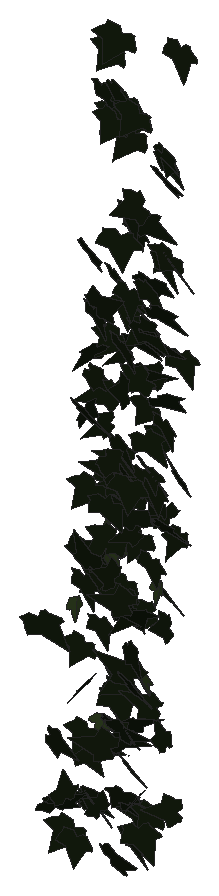
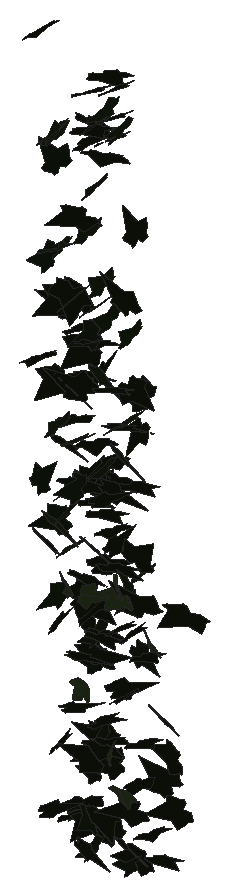
# SketchUp Ruby script. Lengths in inches.
U = 1.inch
M = Sketchup.active_model
def pt(a) = Geom::Point3d.new(a.map { |v| v * U })
def face(e, loops, mat)
  f = e.add_face(loops[0].map { |a| pt(a) })
  loops[1..].each { |l| e.add_face(l.map { |a| pt(a) }).erase! }
  f.material = f.back_material = mat if mat
  f
end
# faces: each face lists its corners as indices into pts; further lists are holes
def faces(e, pts, list, mat = nil) = list.each { |f| face(e, (f[0].is_a?(Array) ? f : [f]).map { |l| l.map { |i| pts[i] } }, mat) }
# xy, xz, yz: faces in a plane at the given z, y or x. An outline is a flat list of corners, or four numbers for a rectangle; further outlines are holes
def ring(l) = l.size == 4 ? [[l[0], l[1]], [l[2], l[1]], [l[2], l[3]], [l[0], l[3]]] : l.each_slice(2).to_a
def flat(e, list, mat, &to3) = list.each { |f| face(e, (f[0].is_a?(Array) ? f : [f]).map { |l| ring(l).map { |u, v| to3.(u, v) } }, mat) }
def xy(e, z, list, mat = nil) = flat(e, list, mat) { |x, y| [x, y, z] }
def xz(e, y, list, mat = nil) = flat(e, list, mat) { |x, z| [x, y, z] }
def yz(e, x, list, mat = nil) = flat(e, list, mat) { |y, z| [x, y, z] }
def lines(e, pts, list) = list.each { |a, b| e.add_line(pt(pts[a]), pt(pts[b])) }
# prism: a flat outline (further loops are holes) pulled along v
def prism(e, loops, v, mat = nil)
  f = face(e, loops, mat); d = Geom::Vector3d.new(v.map { |x| x * U })
  f.pushpull(f.normal.samedirection?(d) ? d.length : -d.length)
end
def box(e, o, s, mat = nil) = prism(e, [[o, [o[0] + s[0], o[1], o[2]], [o[0] + s[0], o[1] + s[1], o[2]], [o[0], o[1] + s[1], o[2]]]], [0, 0, s[2]], mat)
def at(x, y, z, deg = 0) = Geom::Transformation.translation(pt([x, y, z])) * Geom::Transformation.rotation(ORIGIN, Z_AXIS, deg.degrees)
def axes(o, x, y, z) = Geom::Transformation.new([*x, 0, *y, 0, *z, 0, *pt(o).to_a, 1])
def part(name) = M.definitions.add(name)
# library, detail: a bought-in or finely detailed component or shape, given as its bounding box
def library(name, o, s) = part(name).tap { |d| box(d.entities, o, s) }
def detail(e, o, s) = box(e.add_group.entities, o, s)
def put(e, d, t, mat = nil) = e.add_instance(d, t).tap { |i| i.material = mat if mat }
def group(e, t, mat = nil) = e.add_group.tap { |g| g.transformation = t; g.material = mat if mat }.entities
root = M.entities
M.materials.add("1026 AP 7946 SUNNY SIDE UP").color = [254, 231, 186]
M.materials.add("efeu1").color = [18, 25, 13]
M.materials.add("efeu2").color = [43, 57, 29]
c1 = part("ivyleaf_9")
p = [[1.54,2.16,1.25],[1.36,2.04,1.19],[-0.21,0.99,0.68],[-0.71,1.11,0.82],[-0.85,0.86,0.67],[-0.8,0.17,0.21],
  [-0.9,-0.01,0.1],[-0.67,-0.16,-0.02],[-0.08,-0.08,-0.05],[-0.03,-0.6,-0.4],[0.65,-0.88,-0.66],[0.83,-0.6,-0.49],
  [1.29,-0.42,-0.43],[1.8125,-0.07,-0.26],[1.21,0.44,0.15]]
faces(c1.entities,p,[[0,1,2,3,4,5,6,7,8,9,10,11,12,13,14]],"efeu1")
c2 = part("ivyleaf_10")
p = [[0,0.5,-0.03],[-0.0625,2.02,-0.43],[-0.19,2.01,-0.46],[-0.54,1.05,-0.29],[-0.52,0.625,-0.18],[-0.83,0.76,-0.28],
  [-1.16,0.64,-0.33],[-1.15,0.33,-0.24],[-0.77,-0.39,0.02],[-0.3,-0.51,0.16],[0.04,-0.48,0.23],[-0.02,2.01,-0.4375],
  [-0.06,2.01,-0.43],[0.04,-0.49,0.23],[0.67,-0.49,0.14],[1.38,0.36,-0.2],[1.375,0.51,-0.24],[0.81,0.65,-0.19],
  [0.62,0.59,-0.15],[0.6,1.09,-0.28],[0.5,1.23,-0.31]]
faces(c2.entities,p,[[0,1,2,3,4,5,6,7,8,9,10],[11,12,0,13,14,15,16,17,18,19,20]],"efeu2")
put(root,c1,axes([158.63,211.54,302.26],[-0.193,-0.26427,0.31382],[-0.1872,-0.28213,-0.30173],[0.60773,-0.17083,0.00672]),"1026 AP 7946 SUNNY SIDE UP")
put(root,c2,axes([158.375,210.39,301.5],[0.42687,-0.15206,0.25288],[0.29351,-0.16617,-0.31858],[0.34792,0.32675,-0.04151]),"1026 AP 7946 SUNNY SIDE UP")
put(root,c1,axes([158.41,212,299.85],[0.01882,-0.38523,-0.02316],[0.02092,0.0207,-0.39668],[0.60622,0.01125,0.01441]),"1026 AP 7946 SUNNY SIDE UP")
put(root,c1,axes([158.69,212.3,302.82],[-0.28644,-0.2369,0.26948],[-0.16087,-0.24784,-0.30452],[0.53273,-0.20222,0.05294]),"1026 AP 7946 SUNNY SIDE UP")
put(root,c1,axes([158.25,211.11,303.38],[-0.21833,0.04861,0.46385],[0.68202,-0.12015,0.15055],[0.20327,0.45533,-0.00691]),"1026 AP 7946 SUNNY SIDE UP")
put(root,c1,axes([158.86,211.15,313.33],[-0.11675,0.23223,-0.37078],[0.11206,-0.35484,-0.25218],[-0.66589,-0.10043,0.02257]),"1026 AP 7946 SUNNY SIDE UP")
put(root,c2,axes([158.7,211.875,295.34],[0.58802,-0.08102,-0.01424],[-0.03376,-0.03635,-0.39224],[0.12463,0.37243,-0.03908]),"1026 AP 7946 SUNNY SIDE UP")
put(root,c1,axes([158.88,209.57,291.28],[-0.57783,-0.27939,0.06227],[-0.03498,-0.07276,-0.47382],[0.44865,-0.36551,0.04325]),"1026 AP 7946 SUNNY SIDE UP")
put(root,c1,axes([158.34,211,292.09],[0.07738,-0.03027,-0.41689],[0.57726,0.17661,0.03343],[0.27125,-0.36722,0.04778]),"1026 AP 7946 SUNNY SIDE UP")
put(root,c1,axes([158.59,208.22,292.99],[0.03194,0.21488,-0.37217],[0.05224,0.36095,0.22447],[0.66053,-0.03894,0.00024]),"1026 AP 7946 SUNNY SIDE UP")
put(root,c1,axes([158.45,207.96,301.77],[-0.15051,-0.16287,-0.45828],[0.45024,0.34048,-0.1903],[0.5917,-0.30051,0.02824]),"1026 AP 7946 SUNNY SIDE UP")
put(root,c1,axes([158.53,211.29,312.04],[0.41783,-0.28482,-0.21877],[-0.06016,0.23882,-0.38081],[0.55386,0.24081,0.12368]),"1026 AP 7946 SUNNY SIDE UP")
put(root,c1,axes([158.44,211.3,294.39],[0.17299,0.02961,-0.40987],[0.25652,0.37347,0.07726],[0.57276,-0.17621,0.08919]),"1026 AP 7946 SUNNY SIDE UP")
put(root,c1,axes([158.32,208.93,295.69],[0.23693,-0.10053,-0.43884],[0.68673,0.05347,0.14666],[0.02879,-0.44813,0.11315]),"1026 AP 7946 SUNNY SIDE UP")
put(root,c1,axes([158.95,212.25,327.11],[-0.32567,-0.34648,0.24732],[-0.09059,-0.24388,-0.41187],[0.65838,-0.20495,0.06567]),"1026 AP 7946 SUNNY SIDE UP")
put(root,c1,axes([158.59,211.96,325.28],[0.29329,-0.43856,0.06183],[0.01223,-0.06457,-0.491],[0.69646,0.18582,-0.01741]),"1026 AP 7946 SUNNY SIDE UP")
put(root,c2,axes([158.92,211.92,304.68],[0.34785,-0.31239,0.12953],[0.12229,-0.10116,-0.39491],[0.51626,0.23445,0.00627]),"1026 AP 7946 SUNNY SIDE UP")
put(root,c1,axes([159.44,210.62,291.91],[-0.14083,0.19922,0.36869],[-0.32922,0.29125,-0.22],[-0.55173,-0.22464,0.03717]),"1026 AP 7946 SUNNY SIDE UP")
put(root,c1,axes([158.62,211.16,291.87],[0.38671,-0.30197,0.12438],[0.08809,-0.11194,-0.40097],[0.50475,0.2509,-0.02531]),"1026 AP 7946 SUNNY SIDE UP")
put(root,c1,axes([159.15,212.26,313.55],[-0.54377,-0.25492,0.10138],[-0.02444,-0.14234,-0.43062],[0.4298,-0.33061,0.10378]),"1026 AP 7946 SUNNY SIDE UP")
put(root,c1,axes([159.12,210.15,310.93],[-0.01963,-0.03637,-0.45503],[-0.38355,0.36924,-0.02207],[0.58144,0.24234,-0.02992]),"1026 AP 7946 SUNNY SIDE UP")
put(root,c2,axes([158.88,212.37,297.2],[0.01369,-0.1646,0.35889],[0.3275,-0.2922,-0.14891],[0.51127,0.19159,0.08577]),"1026 AP 7946 SUNNY SIDE UP")
put(root,c1,axes([159.19,212.39,327.8],[-0.51356,-0.34852,0.03525],[-0.01394,-0.04125,-0.4918],[0.55078,-0.32601,0.02042]),"1026 AP 7946 SUNNY SIDE UP")
put(root,c1,axes([159.53,211.33,311.34],[-0.5998,-0.0659,0.21862],[-0.27498,-0.17219,-0.37926],[0.21648,-0.40131,0.12398]),"1026 AP 7946 SUNNY SIDE UP")
put(root,c1,axes([159.09,211.98,307.13],[-0.1604,-0.40179,-0.05294],[0.05111,0.04234,-0.42626],[0.63442,-0.105,0.02096]),"1026 AP 7946 SUNNY SIDE UP")
put(root,c1,axes([159.6,211.07,310.07],[-0.58894,0.23093,-0.06474],[0.05545,-0.06464,-0.45215],[-0.37276,-0.37447,0.03503]),"1026 AP 7946 SUNNY SIDE UP")
put(root,c1,axes([158.99,211.19,303.44],[0.15722,-0.36313,0.14132],[0.04607,-0.13632,-0.38874],[0.60979,0.10392,-0.00707]),"1026 AP 7946 SUNNY SIDE UP")
put(root,c1,axes([159.14,210.08,294.875],[0.08827,-0.30312,-0.29422],[-0.06454,0.28101,-0.31584],[0.64981,0.06908,0.0086]),"1026 AP 7946 SUNNY SIDE UP")
put(root,c1,axes([159.02,210.84,315.33],[0.18899,-0.38492,0.19557],[0.07457,-0.18631,-0.4164],[0.67226,0.12888,-0.00879]),"1026 AP 7946 SUNNY SIDE UP")
put(root,c1,axes([159.61,210.33,303.88],[-0.02952,0.29119,0.35933],[-0.01604,0.34708,-0.29847],[-0.71228,-0.01989,-0.00817]),"1026 AP 7946 SUNNY SIDE UP")
put(root,c2,axes([159.26,211.375,303.78],[-0.58108,-0.04479,-0.15772],[0.24827,-0.05235,-0.37779],[0.03286,-0.39647,0.06531]),"1026 AP 7946 SUNNY SIDE UP")
put(root,c1,axes([159.45,209.62,300.22],[-0.35046,-0.32212,0.08648],[-0.05212,-0.08125,-0.40356],[0.52155,-0.22457,0.01777]),"1026 AP 7946 SUNNY SIDE UP")
put(root,c1,axes([159.07,212.1,316.59],[0.32032,-0.37201,0.15364],[0.08346,-0.14317,-0.43725],[0.62591,0.20947,-0.02032]),"1026 AP 7946 SUNNY SIDE UP")
put(root,c1,axes([159.51,211.81,324.42],[-0.3479,-0.32593,0.25349],[-0.08426,-0.25631,-0.39793],[0.63836,-0.21146,0.08562]),"1026 AP 7946 SUNNY SIDE UP")
put(root,c1,axes([159.87,211.92,308.03],[-0.24814,0.02532,0.40139],[-0.5265,-0.22464,-0.12604],[0.31534,-0.35515,0.10541]),"1026 AP 7946 SUNNY SIDE UP")
put(root,c1,axes([159.72,212.05,302.14],[-0.52849,-0.19742,-0.04179],[0.08586,-0.01551,-0.39944],[0.30469,-0.33805,0.04008]),"1026 AP 7946 SUNNY SIDE UP")
put(root,c1,axes([159.66,209.58,296.22],[-0.35773,-0.3412,0.09139],[-0.04162,-0.09105,-0.42203],[0.55355,-0.22735,0.02733]),"1026 AP 7946 SUNNY SIDE UP")
put(root,c1,axes([160.24,210.86,308.13],[-0.23737,-0.08883,-0.43787],[-0.61434,-0.16734,0.17822],[-0.29614,0.41835,-0.01874]),"1026 AP 7946 SUNNY SIDE UP")
put(root,c1,axes([159.91,211.04,304.75],[-0.65537,-0.20291,0.09581],[-0.09333,-0.09165,-0.47469],[0.33912,-0.41736,0.05452]),"1026 AP 7946 SUNNY SIDE UP")
put(root,c1,axes([159.92,209.41,304.24],[0.31097,-0.12589,0.40136],[-0.35368,0.32904,0.22867],[-0.53922,-0.28842,0.08148]),"1026 AP 7946 SUNNY SIDE UP")
put(root,c1,axes([159.55,212.07,297.22],[-0.4124,-0.21599,-0.24334],[0.33465,0.1083,-0.34664],[0.374,-0.33507,0.04184]),"1026 AP 7946 SUNNY SIDE UP")
put(root,c1,axes([159.89,209.7,307.84],[-0.5317,-0.2693,0.06036],[-0.0392,-0.06489,-0.44426],[0.43209,-0.33726,0.03398]),"1026 AP 7946 SUNNY SIDE UP")
put(root,c1,axes([159.46,211.61,325.78],[0.45203,-0.3755,-0.05241],[-0.04078,0.04153,-0.48693],[0.59399,0.28861,0.00645]),"1026 AP 7946 SUNNY SIDE UP")
put(root,c1,axes([159.8,212.25,315.46],[-0.355,-0.35977,-0.0765],[0.18185,0.0107,-0.42736],[0.54759,-0.2368,0.09233]),"1026 AP 7946 SUNNY SIDE UP")
put(root,c2,axes([160.18,212.28,303.92],[0.03925,0.12472,-0.39158],[-0.41255,-0.28331,-0.11496],[-0.47625,0.25569,0.06731]),"1026 AP 7946 SUNNY SIDE UP")
put(root,c1,axes([159.59,207.71,293.53],[0.50354,0.273,-0.06243],[0.03838,0.06684,0.43243],[0.43857,-0.31929,0.03383]),"1026 AP 7946 SUNNY SIDE UP")
put(root,c1,axes([159.95,211.5625,302],[-0.47227,-0.25188,-0.12074],[0.18292,0.04041,-0.40126],[0.39564,-0.31934,0.04139]),"1026 AP 7946 SUNNY SIDE UP")
put(root,c1,axes([160.17,211.51,297.84],[-0.3568,-0.2409,0.29076],[-0.26265,-0.23088,-0.34108],[0.52284,-0.28038,0.02708]),"1026 AP 7946 SUNNY SIDE UP")
put(root,c1,axes([159.81,211.4,297.1],[-0.17577,-0.40182,-0.17373],[0.14838,0.14527,-0.42594],[0.66754,-0.13809,0.04893]),"1026 AP 7946 SUNNY SIDE UP")
put(root,c1,axes([159.76,209.23,303.61],[0.12373,-0.44724,0.05971],[0.00576,-0.06077,-0.46812],[0.70962,0.07847,-0.00661]),"1026 AP 7946 SUNNY SIDE UP")
put(root,c1,axes([159.92,208.56,291.62],[-0.19855,-0.41088,0.013],[0.01253,-0.01809,-0.44273],[0.64637,-0.12586,0.01258]),"1026 AP 7946 SUNNY SIDE UP")
put(root,c1,axes([160.39,211.41,313.63],[-0.51044,0.29772,-0.08286],[0.05277,-0.08443,-0.4525],[-0.48275,-0.32403,0.03815]),"1026 AP 7946 SUNNY SIDE UP")
put(root,c1,axes([159.91,212.03,325.11],[-0.05848,-0.44968,0.12789],[-0.018,-0.12618,-0.46558],[0.73439,-0.0389,-0.00123]),"1026 AP 7946 SUNNY SIDE UP")
put(root,c1,axes([159.62,211,295.98],[0.60817,-0.18434,0.13725],[0.16459,-0.09138,-0.4404],[0.3186,0.3991,-0.03449]),"1026 AP 7946 SUNNY SIDE UP")
put(root,c1,axes([160.15,210.875,324.78],[-0.33681,-0.36204,0.20359],[-0.04085,-0.21265,-0.42716],[0.64883,-0.20132,0.07879]),"1026 AP 7946 SUNNY SIDE UP")
put(root,c1,axes([159.65,209.16,311.61],[0.42336,-0.26869,0.27556],[0.29462,-0.19306,-0.39298],[0.52021,0.328,-0.0017]),"1026 AP 7946 SUNNY SIDE UP")
put(root,c1,axes([159.88,211.27,309.29],[0.32178,-0.37709,-0.02551],[-0.03349,0.01417,-0.44174],[0.59306,0.2054,-0.01111]),"1026 AP 7946 SUNNY SIDE UP")
put(root,c1,axes([160.31,211.18,307.1],[-0.52555,-0.292,0.05395],[-0.02519,-0.06349,-0.456],[0.46625,-0.33257,0.03618]),"1026 AP 7946 SUNNY SIDE UP")
put(root,c1,axes([159.8,210.11,316.07],[-0.08219,0.08953,0.47743],[0.45704,-0.36061,0.10355],[0.58376,0.29494,-0.01385]),"1026 AP 7946 SUNNY SIDE UP")
put(root,c1,axes([159.86,209.45,318.91],[-0.0135,-0.14126,0.46461],[0.27791,-0.42015,-0.13432],[0.69049,0.16634,0.06315]),"1026 AP 7946 SUNNY SIDE UP")
put(root,c1,axes([159.9,212.01,315.68],[0.60451,-0.22304,-0.0106],[-0.02468,-0.00909,-0.45765],[0.35013,0.38445,-0.01396]),"1026 AP 7946 SUNNY SIDE UP")
put(root,c1,axes([160.82,212.23,300.95],[-0.51775,0.0027,0.2258],[-0.33419,-0.10062,-0.32826],[0.08425,-0.38253,0.08555]),"1026 AP 7946 SUNNY SIDE UP")
put(root,c1,axes([160.46,211.85,324.67],[-0.45312,-0.36949,0.04683],[-0.0037,-0.05832,-0.48181],[0.58577,-0.28619,0.03318]),"1026 AP 7946 SUNNY SIDE UP")
put(root,c1,axes([160.51,212.08,304.58],[-0.56101,-0.17067,-0.11801],[0.20164,-0.00792,-0.40277],[0.25151,-0.37435,0.05968]),"1026 AP 7946 SUNNY SIDE UP")
put(root,c1,axes([160.28,210.16,309.07],[0.1949,-0.17801,-0.37693],[-0.06107,0.37456,-0.19965],[0.63544,0.0906,0.09643]),"1026 AP 7946 SUNNY SIDE UP")
put(root,c1,axes([161.04,211.46,291.98],[-0.11962,-0.0545,-0.41965],[-0.63848,-0.05195,0.08505],[-0.09661,0.41082,-0.04244]),"1026 AP 7946 SUNNY SIDE UP")
put(root,c1,axes([160.2,211.36,301.78],[0.41289,-0.36831,0.0219],[-0.01136,-0.03379,-0.46545],[0.58018,0.26145,-0.0247]),"1026 AP 7946 SUNNY SIDE UP")
put(root,c1,axes([160.78,210.6,293.14],[0.31485,0.16325,-0.30777],[-0.34998,-0.2009,-0.26713],[-0.40675,0.29923,-0.00838]),"1026 AP 7946 SUNNY SIDE UP")
put(root,c1,axes([160.39,211.46,316.44],[-0.02217,-0.43747,0.09574],[-0.00509,-0.09537,-0.45147],[0.70404,-0.01446,-0.00025]),"1026 AP 7946 SUNNY SIDE UP")
put(root,c1,axes([160.77,208.23,299.48],[-0.31218,0.28077,-0.26012],[0.1835,-0.22757,-0.35433],[-0.56645,-0.22846,0.02858]),"1026 AP 7946 SUNNY SIDE UP")
put(root,c1,axes([161.11,211.07,305.45],[-0.56809,0.17957,0.01605],[-0.03969,-0.01815,-0.41478],[-0.28049,-0.36112,0.02619]),"1026 AP 7946 SUNNY SIDE UP")
put(root,c1,axes([160.74,212.39,310.66],[-0.32708,-0.29019,0.23698],[-0.00625,-0.2638,-0.34562],[0.58385,-0.16539,0.12906]),"1026 AP 7946 SUNNY SIDE UP")
put(root,c1,axes([160.46,211.25,295.96],[0.27411,0.30839,-0.21995],[0.12762,0.20081,0.36528],[0.57741,-0.19078,0.02368]),"1026 AP 7946 SUNNY SIDE UP")
put(root,c1,axes([161.08,210.99,307.27],[-0.49193,-0.24362,0.14795],[-0.13758,-0.12242,-0.4071],[0.42403,-0.32235,0.03956]),"1026 AP 7946 SUNNY SIDE UP")
put(root,c1,axes([160.66,210.25,295.8],[0.0357,0.12748,-0.43743],[0.06803,0.42323,0.13553],[0.69487,-0.04798,0.00921]),"1026 AP 7946 SUNNY SIDE UP")
put(root,c1,axes([161.13,210.86,324.42],[-0.69989,-0.11343,-0.09335],[0.15094,-0.01349,-0.47182],[0.17042,-0.45391,0.03452]),"1026 AP 7946 SUNNY SIDE UP")
put(root,c1,axes([160.6875,211.51,319.64],[0.0441,-0.36264,0.27513],[0.12083,-0.26188,-0.37331],[0.69972,0.06808,0.04712]),"1026 AP 7946 SUNNY SIDE UP")
put(root,c1,axes([160.78,211.33,314.43],[0.68454,0.09484,0.01284],[0.03144,-0.03596,-0.45743],[-0.14698,0.43402,-0.03803]),"1026 AP 7946 SUNNY SIDE UP")
put(root,c1,axes([161.38,206,295.2],[-0.54665,0.17372,-0.20011],[-0.24649,0.12135,0.39952],[0.32879,0.37981,-0.0332]),"1026 AP 7946 SUNNY SIDE UP")
put(root,c1,axes([161.14,210.53,307.81],[0.47376,-0.21202,0.21313],[-0.19645,0.17845,0.37473],[-0.4238,-0.31974,0.06455]),"1026 AP 7946 SUNNY SIDE UP")
put(root,c1,axes([160.86,209.34,307.62],[-0.2579,-0.23807,-0.32875],[0.36647,0.22061,-0.29292],[0.50545,-0.28143,0.04464]),"1026 AP 7946 SUNNY SIDE UP")
put(root,c1,axes([161.18,210.62,292.73],[0.13548,0.20324,0.34143],[0.14289,0.31832,-0.22436],[-0.59279,0.12318,0.02395]),"1026 AP 7946 SUNNY SIDE UP")
put(root,c1,axes([161.21,210.24,312.43],[-0.09334,-0.0181,0.48812],[-0.32298,-0.42951,-0.04592],[0.67216,-0.2089,0.04572]),"1026 AP 7946 SUNNY SIDE UP")
put(root,c1,axes([161.22,211.81,317.1],[0.57907,0.12079,-0.27461],[-0.3756,-0.12537,-0.39821],[-0.26756,0.43741,-0.03534]),"1026 AP 7946 SUNNY SIDE UP")
put(root,c1,axes([161.52,211.03,312.85],[-0.5695,-0.14385,0.22421],[-0.25781,-0.16586,-0.39353],[0.32046,-0.38909,0.08186]),"1026 AP 7946 SUNNY SIDE UP")
put(root,c1,axes([160.86,210.42,296.42],[0.14366,-0.22161,0.32038],[0.15961,-0.29551,-0.24839],[0.58053,0.13609,-0.01099]),"1026 AP 7946 SUNNY SIDE UP")
put(root,c1,axes([161.34,209.19,304.18],[-0.03578,0.0196,0.46995],[-0.45321,-0.35471,-0.00118],[0.5566,-0.28756,0.02924]),"1026 AP 7946 SUNNY SIDE UP")
put(root,c1,axes([160.6875,210.22,296.23],[0.23867,-0.06949,0.38885],[0.52655,-0.17521,-0.1728],[0.29611,0.36758,-0.00614]),"1026 AP 7946 SUNNY SIDE UP")
put(root,c1,axes([160.83,211.84,308.28],[0.50061,-0.31515,0.08308],[0.05259,-0.08304,-0.46058],[0.50951,0.31822,-0.03409]),"1026 AP 7946 SUNNY SIDE UP")
put(root,c1,axes([161.87,209.74,299.45],[-0.10286,0.09707,0.47598],[-0.68996,0.15814,-0.09742],[-0.27163,-0.43844,0.06722]),"1026 AP 7946 SUNNY SIDE UP")
put(root,c1,axes([161.04,211.7,316.9],[0.27102,-0.38866,-0.16069],[-0.07815,0.1461,-0.43694],[0.65256,0.17891,0.01441]),"1026 AP 7946 SUNNY SIDE UP")
put(root,c1,axes([161.48,211.375,315.08],[-0.39219,-0.26931,0.23706],[-0.16909,-0.21252,-0.37506],[0.53235,-0.26591,0.05551]),"1026 AP 7946 SUNNY SIDE UP")
put(root,c1,axes([161.39,210.8,325.53],[-0.39686,-0.34221,0.19873],[-0.04183,-0.21608,-0.42773],[0.61778,-0.23446,0.0987]),"1026 AP 7946 SUNNY SIDE UP")
put(root,c1,axes([161.67,211.8,312.79],[-0.64091,0.14176,-0.08572],[0.09908,-0.07305,-0.44231],[-0.23942,-0.40971,0.04644]),"1026 AP 7946 SUNNY SIDE UP")
put(root,c1,axes([161.17,210.6,292.67],[0.58662,0.13582,-0.01412],[-0.00492,-0.03361,-0.408],[-0.21472,0.37184,-0.02924]),"1026 AP 7946 SUNNY SIDE UP")
put(root,c1,axes([160.86,211.54,312.53],[0.14238,-0.03928,0.44572],[0.65597,-0.11628,-0.10145],[0.19186,0.42669,0.01609]),"1026 AP 7946 SUNNY SIDE UP")
put(root,c1,axes([161.21,211.33,308.2],[-0.31248,-0.29957,-0.27233],[0.30395,0.18415,-0.36597],[0.54778,-0.27307,0.04771]),"1026 AP 7946 SUNNY SIDE UP")
put(root,c2,axes([161.36,211.01,298.79],[-0.49369,0.20826,-0.12329],[0.13565,-0.08812,-0.38784],[-0.35349,-0.32469,0.02336]),"1026 AP 7946 SUNNY SIDE UP")
put(root,c1,axes([161.12,210.4,291.43],[0.40157,-0.40077,-0.00194],[-0.03106,-0.01305,-0.48904],[0.6294,0.25505,-0.0229]),"1026 AP 7946 SUNNY SIDE UP")
put(root,c1,axes([161.07,210.36,294.78],[0.34475,-0.25292,0.20948],[0.17338,-0.17458,-0.34477],[0.48144,0.24398,-0.02584]),"1026 AP 7946 SUNNY SIDE UP")
put(root,c1,axes([161.23,210.36,321.0625],[0.13691,-0.43626,0.12349],[0.01002,-0.12339,-0.45868],[0.71238,0.08558,-0.01728]),"1026 AP 7946 SUNNY SIDE UP")
put(root,c1,axes([161.13,211.22,320.2],[0.03952,-0.08718,-0.46283],[0.36588,0.38931,-0.06221],[0.61875,-0.22464,0.06635]),"1026 AP 7946 SUNNY SIDE UP")
put(root,c1,axes([161.8,210.15,302.1875],[-0.04549,0.19066,-0.41714],[0.00608,-0.40672,-0.19943],[-0.70525,-0.0158,0.02519]),"1026 AP 7946 SUNNY SIDE UP")
put(root,c1,axes([162.09,209.14,303.15],[-0.23217,-0.015,0.42572],[-0.612,-0.14342,-0.14944],[0.22,-0.41481,0.03355]),"1026 AP 7946 SUNNY SIDE UP")
put(root,c1,axes([162.14,207.89,296.93],[-0.22335,-0.01888,0.46074],[-0.64045,-0.18947,-0.14258],[0.2924,-0.42942,0.03965]),"1026 AP 7946 SUNNY SIDE UP")
put(root,c1,axes([162.13,210.9375,297.54],[-0.28275,-0.31866,-0.16759],[-0.15284,-0.12961,0.37567],[-0.54008,0.20351,-0.01857]),"1026 AP 7946 SUNNY SIDE UP")
put(root,c1,axes([162.07,211.68,310.03],[-0.65182,0.04225,0.00452],[-0.01325,-0.04195,-0.42726],[-0.06543,-0.41243,0.04146]),"1026 AP 7946 SUNNY SIDE UP")
put(root,c1,axes([161.68,211.83,306.73],[-0.15725,-0.24451,0.34814],[-0.08336,-0.33867,-0.26948],[0.65234,-0.10221,0.04949]),"1026 AP 7946 SUNNY SIDE UP")
put(root,c1,axes([161.81,209.83,302.34],[0.46498,0.35482,-0.04409],[-0.01025,-0.05279,-0.47523],[-0.56226,0.29439,-0.0278]),"1026 AP 7946 SUNNY SIDE UP")
put(root,c1,axes([162.31,211.64,306.26],[-0.2697,0.33037,0.17864],[-0.24196,0.10904,-0.37424],[-0.53296,-0.21668,0.0795]),"1026 AP 7946 SUNNY SIDE UP")
put(root,c1,axes([162.19,209.59,306.9],[0.24967,0.06357,0.40614],[-0.61509,0.1082,0.1451],[-0.12342,-0.41066,0.09848]),"1026 AP 7946 SUNNY SIDE UP")
put(root,c1,axes([161.82,211.39,307.62],[0.00308,-0.39988,0.10421],[0.009,-0.10339,-0.41253],[0.6494,0.00333,0.00523]),"1026 AP 7946 SUNNY SIDE UP")
put(root,c1,axes([161.55,208.85,291.07],[0.11016,-0.12082,0.46659],[0.41997,-0.36689,-0.14532],[0.60699,0.27577,0.01587]),"1026 AP 7946 SUNNY SIDE UP")
put(root,c1,axes([162.18,210.77,292.62],[-0.32976,-0.33541,0.14154],[-0.08932,-0.12858,-0.40781],[0.56405,-0.21645,0.01817]),"1026 AP 7946 SUNNY SIDE UP")
put(root,c1,axes([162.12,209.38,308.85],[-0.32781,-0.38001,-0.08054],[0.07326,0.06112,-0.44602],[0.60495,-0.21332,0.01037]),"1026 AP 7946 SUNNY SIDE UP")
put(root,c1,axes([161.73,209.54,299.22],[0.42367,-0.24508,0.227],[0.21763,-0.17612,-0.37483],[0.47191,0.30124,-0.03094]),"1026 AP 7946 SUNNY SIDE UP")
put(root,c1,axes([161.84,209.66,300.78],[-0.10905,-0.0293,-0.45977],[0.69783,-0.05921,-0.06741],[-0.08517,-0.44759,0.03634]),"1026 AP 7946 SUNNY SIDE UP")
put(root,c1,axes([161.97,211.75,310.65],[0.12052,-0.38874,0.16903],[0.06838,-0.16085,-0.40898],[0.6613,0.08748,0.01149]),"1026 AP 7946 SUNNY SIDE UP")
put(root,c1,axes([162.45,211.24,295.79],[-0.2042,-0.32548,0.23568],[0.1374,0.21343,0.36225],[-0.61199,0.15652,0.00269]),"1026 AP 7946 SUNNY SIDE UP")
put(root,c1,axes([162.28,211.87,318.5625],[-0.39861,-0.27139,0.26778],[0.00313,-0.31609,-0.33784],[0.59256,-0.18089,0.18192]),"1026 AP 7946 SUNNY SIDE UP")
put(root,c1,axes([161.89,211.24,316.15],[0.72739,0.02437,0.08263],[0.12901,-0.04329,-0.47503],[-0.02597,0.46748,-0.04553]),"1026 AP 7946 SUNNY SIDE UP")
put(root,c2,axes([162.23,211.07,303.29],[0.43443,-0.27462,0.09348],[0.12068,-0.05361,-0.4013],[0.43927,0.28632,0.0178]),"1026 AP 7946 SUNNY SIDE UP")
put(root,c1,axes([162.01,210.53,310.53],[0.03213,-0.3563,-0.24569],[0.16059,0.23395,-0.35269],[0.65294,-0.04,0.09883]),"1026 AP 7946 SUNNY SIDE UP")
put(root,c1,axes([162.03,211.48,318.57],[0.30299,-0.41095,-0.0027],[-0.02089,-0.00591,-0.46738],[0.64584,0.1926,-0.01385]),"1026 AP 7946 SUNNY SIDE UP")
put(root,c1,axes([162.08,211.45,302.95],[0.54057,-0.22096,-0.07817],[-0.0996,0.03947,-0.42078],[0.35293,0.34957,0.00099]),"1026 AP 7946 SUNNY SIDE UP")
put(root,c1,axes([162.03,208.86,315.69],[0.19823,-0.39312,0.23963],[0.12102,-0.22193,-0.42657],[0.7098,0.14763,0.0058]),"1026 AP 7946 SUNNY SIDE UP")
put(root,c1,axes([162.18,210.72,304.61],[0.00959,-0.40269,0.12179],[0.04629,-0.11981,-0.4147],[0.65932,0.01427,0.02735]),"1026 AP 7946 SUNNY SIDE UP")
put(root,c1,axes([162.62,209.42,322.14],[-0.33181,-0.19692,0.39714],[-0.34668,-0.32161,-0.29461],[0.58759,-0.30096,0.05045]),"1026 AP 7946 SUNNY SIDE UP")
put(root,c1,axes([162.52,211.37,301.25],[-0.1428,-0.09618,0.41684],[-0.27013,-0.36911,-0.13209],[0.59648,-0.19019,0.03997]),"1026 AP 7946 SUNNY SIDE UP")
put(root,c1,axes([162.01,210.24,315.95],[-0.00367,-0.08355,-0.47099],[0.69824,0.13297,-0.02662],[0.21318,-0.43694,0.07908]),"1026 AP 7946 SUNNY SIDE UP")
put(root,c1,axes([162.36,211.56,323.46],[-0.06652,-0.31906,0.34369],[0.06307,-0.33808,-0.32806],[0.72519,0.00014,0.06005]),"1026 AP 7946 SUNNY SIDE UP")
put(root,c1,axes([162.16,211.19,306.15],[0.59537,-0.09402,0.11444],[0.17449,-0.01608,-0.40186],[0.14903,0.39442,0.01334]),"1026 AP 7946 SUNNY SIDE UP")
put(root,c1,axes([162.79,211.98,307.87],[0.21239,-0.32845,0.29332],[-0.14845,0.27087,0.36723],[-0.66914,-0.16434,0.01163]),"1026 AP 7946 SUNNY SIDE UP")
put(root,c1,axes([162.15,211.53,322.32],[0.0735,-0.23173,0.42884],[0.348,-0.3613,-0.23418],[0.66544,0.21454,0.0751]),"1026 AP 7946 SUNNY SIDE UP")
put(root,c1,axes([162.19,211.94,318.3],[0.45985,-0.32695,0.11846],[0.07262,-0.11478,-0.45063],[0.54109,0.29327,-0.04019]),"1026 AP 7946 SUNNY SIDE UP")
put(root,c1,axes([162.69,211.91,305.5],[-0.55331,-0.00571,-0.23034],[0.34647,-0.08006,-0.35566],[-0.06008,-0.40914,0.07032]),"1026 AP 7946 SUNNY SIDE UP")
put(root,c1,axes([162.42,210.94,312.28],[0.52804,0.24794,0.10896],[0.16565,0.03238,-0.42829],[-0.3892,0.35017,-0.03445]),"1026 AP 7946 SUNNY SIDE UP")
put(root,c1,axes([162.98,211.26,292.72],[-0.27475,-0.08164,0.3927],[-0.4758,-0.23577,-0.19606],[0.38761,-0.34729,0.0377]),"1026 AP 7946 SUNNY SIDE UP")
put(root,c1,axes([162.52,208.23,321.2],[-0.40248,-0.34593,-0.19796],[0.29475,0.09299,-0.43358],[0.5463,-0.30504,0.08808]),"1026 AP 7946 SUNNY SIDE UP")
put(root,c1,axes([162.375,211.27,323.67],[0.3588,-0.39326,-0.0949],[-0.06914,0.07841,-0.46793],[0.63052,0.23238,0.00269]),"1026 AP 7946 SUNNY SIDE UP")
put(root,c1,axes([162.55,212.22,313.82],[-0.02294,-0.42327,-0.1031],[0.0748,0.09558,-0.43349],[0.67894,-0.02484,0.04428]),"1026 AP 7946 SUNNY SIDE UP")
put(root,c1,axes([162.58,209.41,292.54],[-0.11447,-0.39933,-0.26055],[0.07084,0.24656,-0.41672],[0.73795,-0.08561,-0.00041]),"1026 AP 7946 SUNNY SIDE UP")
put(root,c1,axes([162.65,212.07,328.48],[-0.03702,-0.47874,0.04666],[-0.01209,-0.04769,-0.49404],[0.75645,-0.02419,-0.00561]),"1026 AP 7946 SUNNY SIDE UP")
put(root,c1,axes([162.37,210.33,315.26],[0.35045,-0.13158,0.38174],[0.47823,-0.21365,-0.26732],[0.39366,0.37669,-0.01509]),"1026 AP 7946 SUNNY SIDE UP")
